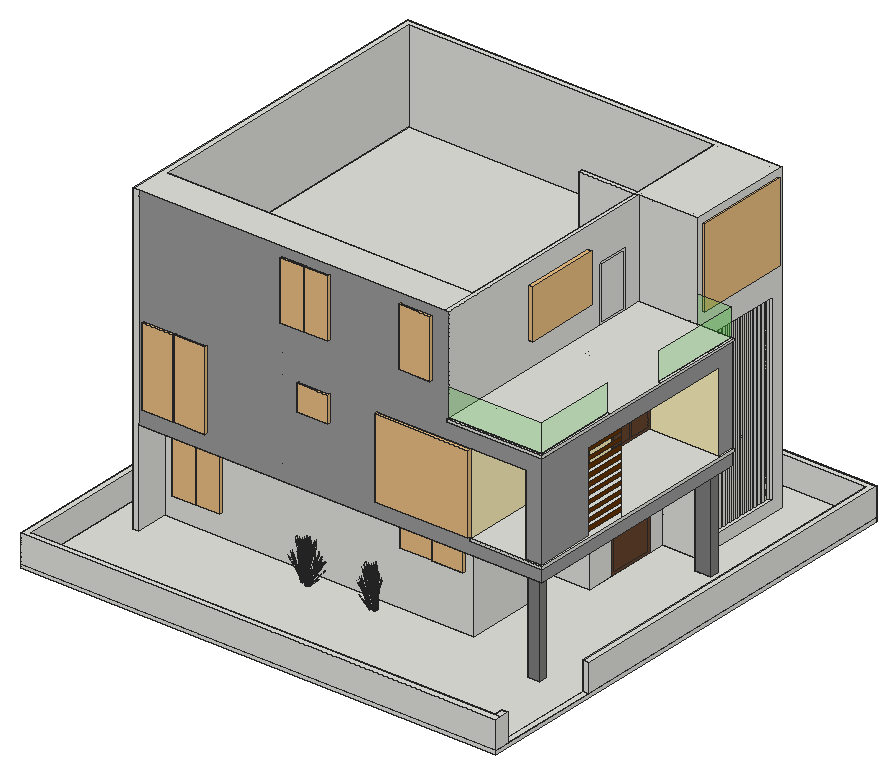
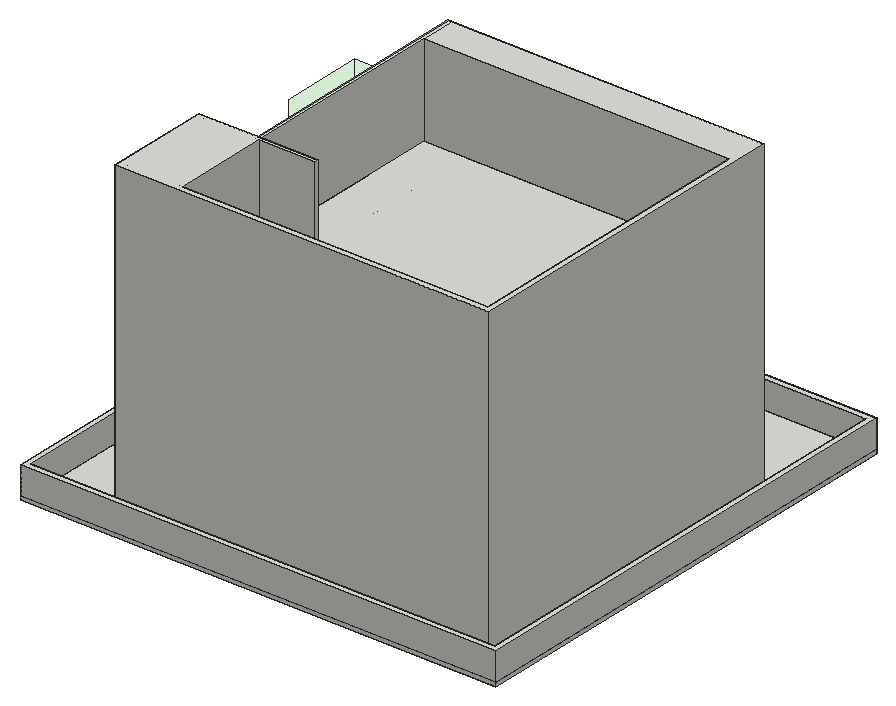
# SketchUp Ruby script. Lengths in millimetres.
U = 1.mm
M = Sketchup.active_model
def pt(a) = Geom::Point3d.new(a.map { |v| v * U })
def face(e, loops, mat)
  f = e.add_face(loops[0].map { |a| pt(a) })
  loops[1..].each { |l| e.add_face(l.map { |a| pt(a) }).erase! }
  f.material = f.back_material = mat if mat
  f
end
# faces: each face lists its corners as indices into pts; further lists are holes
def faces(e, pts, list, mat = nil) = list.each { |f| face(e, (f[0].is_a?(Array) ? f : [f]).map { |l| l.map { |i| pts[i] } }, mat) }
# xy, xz, yz: faces in a plane at the given z, y or x. An outline is a flat list of corners, or four numbers for a rectangle; further outlines are holes
def ring(l) = l.size == 4 ? [[l[0], l[1]], [l[2], l[1]], [l[2], l[3]], [l[0], l[3]]] : l.each_slice(2).to_a
def flat(e, list, mat, &to3) = list.each { |f| face(e, (f[0].is_a?(Array) ? f : [f]).map { |l| ring(l).map { |u, v| to3.(u, v) } }, mat) }
def xy(e, z, list, mat = nil) = flat(e, list, mat) { |x, y| [x, y, z] }
def xz(e, y, list, mat = nil) = flat(e, list, mat) { |x, z| [x, y, z] }
def yz(e, x, list, mat = nil) = flat(e, list, mat) { |y, z| [x, y, z] }
def lines(e, pts, list) = list.each { |a, b| e.add_line(pt(pts[a]), pt(pts[b])) }
# prism: a flat outline (further loops are holes) pulled along v
def prism(e, loops, v, mat = nil)
  f = face(e, loops, mat); d = Geom::Vector3d.new(v.map { |x| x * U })
  f.pushpull(f.normal.samedirection?(d) ? d.length : -d.length)
end
def box(e, o, s, mat = nil) = prism(e, [[o, [o[0] + s[0], o[1], o[2]], [o[0] + s[0], o[1] + s[1], o[2]], [o[0], o[1] + s[1], o[2]]]], [0, 0, s[2]], mat)
def at(x, y, z, deg = 0) = Geom::Transformation.translation(pt([x, y, z])) * Geom::Transformation.rotation(ORIGIN, Z_AXIS, deg.degrees)
def axes(o, x, y, z) = Geom::Transformation.new([*x, 0, *y, 0, *z, 0, *pt(o).to_a, 1])
def part(name) = M.definitions.add(name)
# library, detail: a bought-in or finely detailed component or shape, given as its bounding box
def library(name, o, s) = part(name).tap { |d| box(d.entities, o, s) }
def detail(e, o, s) = box(e.add_group.entities, o, s)
def put(e, d, t, mat = nil) = e.add_instance(d, t).tap { |i| i.material = mat if mat }
def group(e, t, mat = nil) = e.add_group.tap { |g| g.transformation = t; g.material = mat if mat }.entities
root = M.entities
M.materials.add("C08_Toffee_Ember").color = [102, 51, 0]
M.materials.add("D02_Buttercup_Glow").color = [255, 242, 189]
M.materials.add("Glass_Basic_01").color = [75, 255, 58]
M.materials["Glass_Basic_01"].alpha = 0.2
M.materials.add("LightPink_Translucent").color = [144, 107, 117]
M.materials["LightPink_Translucent"].alpha = 0.8
M.materials.add("ThomThom - Waistcoat1").color = [155, 155, 155]
M.materials.add("ThomThom - Waistcoat2").color = [127, 127, 126]
M.materials.add("Wood_Veneer_15_1K").color = [103, 69, 45]
c1 = part("blade")
p = [[54.7,5.3,558.8],[0,4.4,0],[2.3,11.5,0],[55.5,7.8,558.8],[58.2,7.8,558.8],[9.8,11.5,0],
  [62.9,5.7,838.2],[63,6,838.2],[63.4,6,838.2]]
faces(c1.entities,p,[[0,1,2,3],[4,5,2,3],[6,0,3,7],[7,3,4,8]])
c2 = part("seeds")
p = [[7.6,-2.7,35.1],[-0.2,-0.6,40.4],[-0.2,-0.8,0.9],[3.5,-1.8,-1.7],[7.5,-0.8,76.3],[3.7,0.2,78.9]]
faces(c2.entities,p,[[0,1,2,3],[1,0,4,5]],"LightPink_Translucent")
c3 = part("blade with seeds")
put(c3.entities,c1,at(0,0,0))
put(c3.entities,c2,axes([60.9,6.5,787.2],[1.5799,-0.05474,1.17369],[-0.12525,1.92788,0.29478],[-0.07173,-0.02425,1.56792]))
c4 = library("Three-panel window",[0,0,0],[127.5,2149.6,1524])
c5 = library("Group\#4",[0,0,0],[1200.6,88.7,3023])
put(root,c3,axes([7561.3,4255.6,60.5],[-1.54892,-0.2182,0.49198],[0.31522,-1.23236,0.19306],[0.22636,0.119,1.70813]))
put(root,c3,axes([9992.7,4305.7,37.9],[0.03108,0.16322,1.76342],[-0.62654,0.85237,-0.26939],[-0.44504,-0.04296,0.30037]))
put(root,c3,axes([7529.9,4332.9,56],[-0.39985,-0.89288,0],[1.1418,-0.31268,0],[0,0,1.54371]))
put(root,c3,axes([7510.5,4311.4,66.5],[-0.23642,0.92427,0.1448],[-1.15506,-0.16044,-0.41347],[-0.21021,-0.09491,1.26744]))
put(root,c3,axes([10062.4,4383.8,51.5],[-0.28787,-0.90242,-0.30978],[1.14332,-0.25625,0.30978],[-0.23049,-0.10406,1.38974]))
put(root,c3,axes([7567.9,4329.7,55.5],[1.2866,-0.3514,-0.19198],[0.45209,1.01223,0.00008],[0.14202,-0.03884,1.73897]))
put(root,c3,axes([7579.2,4340.5,62.8],[0.35402,-1.02926,0.17642],[1.29548,0.29127,0.35086],[-0.22379,0.00501,1.60407]))
put(root,c3,axes([7571.7,4281.2,56.2],[0.85545,0.66896,0],[-0.85545,0.66896,0],[0,0,1.69266]))
put(root,c3,axes([10099.7,4382.5,62.8],[1.31687,-0.27488,0.17642],[0.32517,1.02297,0.35086],[-0.11745,-0.14905,1.60407]))
put(root,c3,axes([7448.2,4249.3,84.9],[0.34834,-0.14982,1.77064],[0.12012,1.04605,0.13857],[-0.75452,0.1388,0.63284]))
put(root,c3,axes([7630.6,4273.8,62.8],[-0.96285,-0.75439,0.17642],[0.97031,-0.7317,0.35086],[-0.10634,0.15406,1.60407]))
put(root,c3,axes([7585.3,4244.8,52.3],[1.27479,0.1698,-0.62353],[-0.26901,1.04736,-0.16365],[0.38043,0.12691,1.37633]))
put(root,c3,axes([10054.3,4393.7,51.2],[-1.14694,-0.51783,-0.49651],[0.68554,-0.92854,0],[-0.26122,-0.11794,1.57504]))
put(root,c3,axes([7728.4,4291.3,70.2],[-0.75718,0.17097,1.1486],[0.35641,-0.70661,0.84392],[0.40168,0.04835,0.25299]))
put(root,c3,axes([9989.4,4296.3,115],[-1.01846,-0.28891,-0.35414],[0.29705,-0.84289,0.4572],[-0.41005,0.07729,0.87481]))
put(root,c3,axes([7522.7,4343.2,55.8],[-1.23546,-0.46496,0],[0.59459,-0.96613,0],[0,0,1.62707]))
put(root,c3,axes([7548.8,4311.7,62.6],[-1.19666,-0.83357,-0.25192],[1.00694,-0.93603,0.5513],[-0.32224,0.09751,1.68216]))
put(root,c3,axes([7468.8,4352.3,63],[1.14694,0.51783,0.49651],[-0.68554,0.92854,0],[-0.26122,-0.11794,1.57504]))
put(root,c3,axes([10133.5,4347.2,67.7],[-1.23732,0.68758,-0.29095],[-0.8228,-0.97154,-0.50002],[-0.30528,-0.09867,1.59708]))
put(root,c3,axes([7571.5,4261.3,69],[0.59459,-0.93321,0.44739],[1.23546,0.44912,-0.21531],[0,0.21512,1.43643]))
put(root,c3,axes([7565.7,4274.8,58.2],[0,1.19774,-0.05637],[-1.53239,0,0],[0,0.03764,1.79368]))
put(root,c3,axes([7387.2,4263.8,118.9],[-0.332,0.94205,-0.51099],[-1.13828,-0.3229,-0.3958],[-0.45829,0.08638,0.97773]))
put(root,c3,axes([7568.5,4253.3,56.2],[0.73619,0.86927,-0.44739],[-1.11511,0.61213,0.21531],[0.23824,0.10756,1.43643]))
put(root,c3,axes([7695,4346.6,99.8],[-0.23455,-0.87059,-0.03492],[1.10861,-0.20015,-0.15832],[0.23151,0.05519,0.52218]))
put(root,c3,axes([7452,4366.1,60.3],[-0.7662,1.03778,0],[-1.28187,-0.57875,-0.51607],[-0.29196,-0.13181,1.63711]))
put(root,c3,axes([10130.5,4354.9,66.5],[-0.23642,0.92427,0.1448],[-1.15506,-0.16044,-0.41347],[-0.21021,-0.09491,1.26744]))
put(root,c3,axes([7650.7,4274.5,63],[0,-1.03566,0.49651],[1.37109,0,0],[0,0.23588,1.57504]))
put(root,c3,axes([7563.5,4294.2,69],[1.33077,-0.06393,0.44739],[0.12035,1.06125,-0.21531],[-0.23824,0.10756,1.43643]))
put(root,c3,axes([7584.6,4266.7,66.5],[1.1418,-0.30203,0.1448],[0.39985,0.86246,-0.41347],[0,0.18981,1.26744]))
put(root,c3,axes([10199.2,4383.9,62.8],[0.35402,-1.02926,0.17642],[1.29548,0.29127,0.35086],[-0.22379,0.00501,1.60407]))
put(root,c3,axes([7533.4,4307.2,56.2],[-1.33077,0.06393,-0.44739],[-0.12035,-1.06125,0.21531],[-0.23824,0.10756,1.43643]))
put(root,c3,axes([10068.2,4292.7,84.9],[0.34834,-0.14982,1.77064],[0.12012,1.04605,0.13857],[-0.75452,0.1388,0.63284]))
put(root,c3,axes([7692.3,4320.1,65.8],[-0.29514,-0.25472,1.43002],[0.38401,-0.84262,-0.30754],[0.59714,0.11414,0.61141]))
put(root,c3,axes([10142.7,4386.6,55.8],[-1.23546,-0.46496,0],[0.59459,-0.96613,0],[0,0,1.62707]))
put(root,c3,axes([10168.8,4355.2,62.6],[-1.19666,-0.83357,-0.25192],[1.00694,-0.93603,0.5513],[-0.32224,0.09751,1.68216]))
put(root,c3,axes([10088.8,4395.8,63],[1.14694,0.51783,0.49651],[-0.68554,0.92854,0],[-0.26122,-0.11794,1.57504]))
put(root,c3,axes([7558.3,4343.6,56],[1.23546,0.46496,0],[-0.59459,0.96613,0],[0,0,1.74954]))
put(root,c3,axes([7570.9,4369.7,55.7],[-0.75665,-1.04141,-0.05142],[1.28187,-0.57875,0.51607],[-0.31588,0.09915,1.6363]))
put(root,c3,axes([7564,4305.8,66.5],[0.90538,0.62224,0.1448],[-0.75521,0.70202,-0.41347],[-0.21021,0.09491,1.26744]))
put(root,c3,axes([7386.2,4276.1,98.5],[0.42521,-0.21906,1.71376],[0.35798,1.01226,0.13857],[-0.66754,0.22878,0.73262]))
put(root,c3,axes([10007.2,4307.2,118.9],[-0.332,0.94205,-0.51099],[-1.13828,-0.3229,-0.3958],[-0.45829,0.08638,0.97773]))
put(root,c3,axes([10072,4409.5,60.3],[-0.7662,1.03778,0],[-1.28187,-0.57875,-0.51607],[-0.29196,-0.13181,1.63711]))
put(root,c3,axes([10183.5,4337.6,69],[1.33077,-0.06393,0.44739],[0.12035,1.06125,-0.21531],[-0.23824,0.10756,1.43643]))
put(root,c3,axes([7623.5,4333.1,126.5],[1.22504,0.02494,-0.71045],[-0.08228,1.05005,0.08574],[0.51899,0.11081,1.00501]))
put(root,c3,axes([7588.5,4354.5,63],[1.14694,-0.51783,0.49651],[0.68554,0.92854,0],[-0.26122,0.11794,1.57504]))
put(root,c3,axes([10153.4,4350.7,56.2],[-1.33077,0.06393,-0.44739],[-0.12035,-1.06125,0.21531],[-0.23824,0.10756,1.43643]))
put(root,c3,axes([7547.1,4333.7,58.2],[0.53281,1.18979,-0.06012],[-1.52239,0.41691,0],[0.01861,0.04155,1.72173]))
put(root,c3,axes([7562.1,4366.4,51.5],[-1.14332,-0.25625,-0.30978],[0.28787,-0.90242,0.30978],[-0.23049,0.10406,1.38974]))
put(root,c3,axes([7352.5,4319.9,65.8],[0.42589,0.08502,1.43002],[0.2745,0.86839,-0.30754],[-0.57851,0.16255,0.61141]))
put(root,c3,axes([7674.4,4279,60.4],[1.53239,0,0],[0,1.1575,-0.51607],[0,0.26363,1.63711]))
put(root,c3,axes([7658.8,4294.1,55.9],[-1.53164,-0.00828,-0.04976],[0,-1.1575,0.49943],[-0.04813,0.2635,1.58352]))
put(root,c3,axes([7574.6,4268.5,67.7],[1.38012,0.49416,-0.29095],[-0.66454,1.04299,-0.50002],[0.04337,0.25608,1.59708]))
put(root,c3,axes([7330,4366.1,70.2],[0.51072,-0.46938,1.1486],[0.20153,0.74307,0.84392],[-0.36908,0.13305,0.25299]))
put(root,c3,axes([7642.2,4344.1,115],[0.69728,0.64842,-0.35414],[-0.79619,0.61382,0.4572],[0.40453,0.09339,0.87481]))
put(root,c3,axes([7650.7,4298.3,51.5],[-0.85545,0.64616,-0.30978],[-0.85545,-0.64616,0.30978],[0,0.20813,1.38974]))
put(root,c3,axes([7557.1,4299.9,67.7],[0.1428,1.18174,-0.29095],[-1.48733,0.07145,-0.50002],[-0.26191,0.15741,1.59708]))
put(root,c3,axes([10190.8,4413.2,55.7],[-0.75665,-1.04141,-0.05142],[1.28187,-0.57875,0.51607],[-0.31588,0.09915,1.6363]))
put(root,c3,axes([7570.9,4288.2,56.2],[-0.59459,0.93321,-0.44739],[-1.23546,-0.44912,0.21531],[0,0.21512,1.43643]))
put(root,c3,axes([10184,4349.2,66.5],[0.90538,0.62224,0.1448],[-0.75521,0.70202,-0.41347],[-0.21021,0.09491,1.26744]))
put(root,c3,axes([7378.9,4314.6,115],[-1.06674,0.14801,-0.35414],[-0.28168,-0.84611,0.4572],[-0.30569,0.22726,0.87481]))
put(root,c3,axes([10006.2,4319.5,98.5],[0.42521,-0.21906,1.71376],[0.35798,1.01226,0.13857],[-0.66754,0.22878,0.73262]))
put(root,c3,axes([7534.4,4322.9,52.3],[-0.82544,0.77843,-0.62353],[-1.0254,-0.70586,-0.16365],[-0.33076,0.19418,1.37633]))
put(root,c3,axes([10208.5,4397.9,63],[1.14694,-0.51783,0.49651],[0.68554,0.92854,0],[-0.26122,0.11794,1.57504]))
put(root,c3,axes([10182.1,4409.9,51.5],[-1.14332,-0.25625,-0.30978],[0.28787,-0.90242,0.30978],[-0.23049,0.10406,1.38974]))
put(root,c3,axes([7571.7,4356.2,59.2],[1.53422,0.33662,0.30756],[-0.38383,1.20322,-0.36492],[-0.25393,0.15059,1.64885]))
put(root,c3,axes([7568.9,4376.8,51.2],[-1.14694,0.51783,-0.49651],[-0.68554,-0.92854,0],[-0.26122,0.11794,1.57504]))
put(root,c3,axes([7665.7,4298.9,51.2],[0,1.03566,-0.49651],[-1.37109,0,0],[0,0.23588,1.57504]))
put(root,c3,axes([9972.5,4363.4,65.8],[0.42589,0.08502,1.43002],[0.2745,0.86839,-0.30754],[-0.57851,0.16255,0.61141]))
put(root,c3,axes([7578.6,4301.9,98.5],[-0.45521,-0.17844,1.71376],[0.94204,-0.74856,0.13857],[0.58713,0.33769,0.73262]))
put(root,c3,axes([9950,4409.6,70.2],[0.51072,-0.46938,1.1486],[0.20153,0.74307,0.84392],[-0.36908,0.13305,0.25299]))
put(root,c3,axes([7621.4,4353.5,70.2],[-0.69001,-0.29779,1.1486],[0.89096,-0.30257,0.84392],[0.24031,0.2563,0.25299]))
put(root,c3,axes([10177.1,4343.4,67.7],[0.1428,1.18174,-0.29095],[-1.48733,0.07145,-0.50002],[-0.26191,0.15741,1.59708]))
put(root,c3,axes([9998.9,4358,115],[-1.06674,0.14801,-0.35414],[-0.28168,-0.84611,0.4572],[-0.30569,0.22726,0.87481]))
put(root,c3,axes([7425.7,4293.4,98.5],[0.30609,-0.31822,1.71376],[0.77286,0.85893,0.13857],[-0.53009,0.39116,0.73262]))
put(root,c3,axes([7401.3,4317.1,118.9],[0.31482,0.94565,-0.51099],[-1.19224,0.16542,-0.3958],[-0.34166,0.254,0.97773]))
put(root,c3,axes([7595.3,4372.7,60.3],[0.7662,1.03778,0],[-1.28187,0.57875,-0.51607],[-0.29196,0.13181,1.63711]))
put(root,c3,axes([7626.4,4381.6,37.9],[0.08928,-0.14952,1.76342],[1.12407,-0.44035,-0.26939],[0.34078,0.22791,0.30037]))
put(root,c3,axes([7578.8,4268.4,72.2],[-0.03348,-0.97511,1.41272],[1.51511,0.25277,0.59816],[-0.35835,0.53357,1.3335]))
put(root,c3,axes([7588.6,4295.3,53.2],[0.44936,0.94823,-0.69212],[-1.29441,0.3415,-0.18165],[0.04967,0.32109,1.52773]))
put(root,c3,axes([10154.4,4366.3,52.3],[-0.82544,0.77843,-0.62353],[-1.0254,-0.70586,-0.16365],[-0.33076,0.19418,1.37633]))
put(root,c3,axes([7364.1,4378.4,37.9],[0.16438,0.10347,1.76342],[0.27873,0.95868,-0.26939],[-0.36432,0.20444,0.30037]))
put(root,c3,axes([7581.8,4363.9,118.9],[1.20928,-0.24619,-0.51099],[0.21154,0.93233,-0.3958],[0.32481,0.26718,0.97773]))
put(root,c3,axes([10191.7,4399.6,59.2],[1.53422,0.33662,0.30756],[-0.38383,1.20322,-0.36492],[-0.25393,0.15059,1.64885]))
put(root,c3,axes([10188.9,4420.3,51.2],[-1.14694,0.51783,-0.49651],[-0.68554,-0.92854,0],[-0.26122,0.11794,1.57504]))
put(root,c3,axes([7624.2,4387.9,67.7],[-0.78586,-0.03248,1.0506],[0.51898,-0.68985,0.58006],[0.31045,0.24509,0.8241]))
put(root,c3,axes([10045.7,4336.9,98.5],[0.30609,-0.31822,1.71376],[0.77286,0.85893,0.13857],[-0.53009,0.39116,0.73262]))
put(root,c3,axes([10021.3,4360.5,118.9],[0.31482,0.94565,-0.51099],[-1.19224,0.16542,-0.3958],[-0.34166,0.254,0.97773]))
put(root,c3,axes([7419.9,4313.3,98.5],[0.22818,-0.35597,1.71376],[0.95725,0.73667,0.13857],[-0.43183,0.45914,0.73262]))
put(root,c3,axes([10215.3,4416.2,60.3],[0.7662,1.03778,0],[-1.28187,0.57875,-0.51607],[-0.29196,0.13181,1.63711]))
put(root,c3,axes([7559.1,4345.4,65.8],[0.02163,-0.34331,1.43002],[1.03345,-0.38348,-0.30754],[0.31903,0.4109,0.61141]))
put(root,c3,axes([10198.7,4311.8,72.2],[-0.03348,-0.97511,1.41272],[1.51511,0.25277,0.59816],[-0.35835,0.53357,1.3335]))
put(root,c3,axes([9984.1,4421.8,37.9],[0.16438,0.10347,1.76342],[0.27873,0.95868,-0.26939],[-0.36432,0.20444,0.30037]))
put(root,c3,axes([7426.6,4364.3,115],[-0.82919,0.54528,-0.35414],[-0.78493,-0.62262,0.4572],[-0.11943,0.31634,0.87481]))
put(root,c3,axes([7440,4418.1,70.2],[-0.03171,-0.6158,1.1486],[0.7925,0.43922,0.84392],[-0.15586,0.29352,0.25299]))
put(root,c3,axes([7493,4380.8,37.9],[0.19833,-0.05635,1.76342],[1.19302,0.31018,-0.26939],[0.03489,0.3496,0.30037]))
put(root,c3,axes([7447.5,4357.8,127.1],[0.87728,0.69587,-0.5672],[-0.92674,0.60943,-0.43934],[-0.13348,0.35356,1.08528]))
put(root,c3,axes([7423.3,4384.3,71.7],[1.11329,-0.1834,0.06507],[0.25594,0.73887,-0.86304],[-0.07058,0.37403,0.7736]))
put(root,c3,axes([7513.6,4374.9,118.9],[1.20468,0.25962,-0.51099],[-0.41292,0.89013,-0.3958],[0.11046,0.35838,0.97773]))
put(root,c3,axes([7531,4328.2,98.5],[-0.28013,-0.33252,1.71376],[1.29445,-0.27994,0.13857],[0.29256,0.52202,0.73262]))
put(root,c3,axes([10039.9,4356.8,98.5],[0.22818,-0.35597,1.71376],[0.95725,0.73667,0.13857],[-0.43183,0.45914,0.73262]))
put(root,c3,axes([7499.7,4388.8,115],[-0.36946,0.79643,-0.35414],[-1.07787,-0.23229,0.4572],[0.09883,0.32066,0.87481]))
put(root,c3,axes([10046.6,4407.8,115],[-0.82919,0.54528,-0.35414],[-0.78493,-0.62262,0.4572],[-0.11943,0.31634,0.87481]))
put(root,c3,axes([7440.6,4349.7,135.6],[-0.03189,0.95798,-0.7886],[-1.34277,-0.06434,0.09517],[-0.14171,0.40585,1.11556]))
put(root,c3,axes([10060,4461.6,70.2],[-0.03171,-0.6158,1.1486],[0.7925,0.43922,0.84392],[-0.15586,0.29352,0.25299]))
put(root,c3,axes([7472.9,4332.4,98.5],[-0.02999,-0.3975,1.71376],[1.30002,0.26369,0.13857],[-0.08041,0.56647,0.73262]))
put(root,c3,axes([7502.5,4370.6,126.5],[0.5849,0.8421,-0.71045],[-1.20401,0.4693,0.08574],[0.13677,0.40688,1.00501]))
put(root,c3,axes([10067.5,4401.2,127.1],[0.87728,0.69587,-0.5672],[-0.92674,0.60943,-0.43934],[-0.13348,0.35356,1.08528]))
put(root,c3,axes([7416.5,4404.3,65.8],[0.38672,-0.16338,1.43002],[0.95481,0.49262,-0.30754],[-0.28419,0.42626,0.61141]))
put(root,c3,axes([10043.3,4427.8,71.7],[1.11329,-0.1834,0.06507],[0.25594,0.73887,-0.86304],[-0.07058,0.37403,0.7736]))
put(root,c3,axes([10060.6,4393.1,135.6],[-0.03189,0.95798,-0.7886],[-1.34277,-0.06434,0.09517],[-0.14171,0.40585,1.11556]))
put(root,c3,axes([10092.9,4375.9,98.5],[-0.02999,-0.3975,1.71376],[1.30002,0.26369,0.13857],[-0.08041,0.56647,0.73262]))
put(root,c3,axes([7429.2,4384,85.4],[0.02693,-0.53464,1.54345],[1.21102,0.2824,0.21329],[-0.10493,0.5698,0.72882]))
put(root,c3,axes([10036.5,4447.7,65.8],[0.38672,-0.16338,1.43002],[0.95481,0.49262,-0.30754],[-0.28419,0.42626,0.61141]))
put(root,c3,axes([10049.2,4427.4,85.4],[0.02693,-0.53464,1.54345],[1.21102,0.2824,0.21329],[-0.10493,0.5698,0.72882]))
g1 = group(root,at(0,0,-152.4))
xy(g1,0,[[0,0,18288,18288]])
xy(g1,152.4,[[228.6,228.6,18059.4,18059.4],[18059.4,562.7,18288,4460.6]])
xy(g1,1219.2,[[0,0,18288,0,18288,228.6,228.6,228.6,228.6,18059.4,18059.4,18059.4,18059.4,4460.6,18288,4460.6,18288,18288,0,18288],[18059.4,228.6,18288,562.7]])
xz(g1,0,[[0,0,18288,1219.2]])
xz(g1,228.6,[[228.6,152.4,18059.4,1219.2]])
xz(g1,562.7,[[18059.4,152.4,18288,1219.2]])
xz(g1,4460.6,[[18059.4,152.4,18288,1219.2]])
xz(g1,18059.4,[[228.6,152.4,18059.4,1219.2]])
xz(g1,18288,[[0,0,18288,1219.2]])
yz(g1,0,[[0,0,18288,1219.2]])
yz(g1,228.6,[[228.6,152.4,18059.4,1219.2]])
yz(g1,18059.4,[[228.6,152.4,562.7,1219.2],[4460.6,152.4,11604.7,1219.2],[11604.7,152.4,18059.4,1219.2]])
yz(g1,18288,[[0,0,18288,0,18288,1219.2,4460.6,1219.2,4460.6,152.4,562.7,152.4,562.7,1219.2,0,1219.2]])
g2 = group(root,at(0,0,0))
xy(g2,0,[[1295.4,3810,1524,3810,1524,5029.2,13411.2,5029.2,13411.2,5181.6,1524,5181.6,1524,16764,14173.2,16764,14173.2,9448.8,14325.6,9448.8,14325.6,16764,15392.4,16764,15392.4,12954,15544.8,12954,15544.8,16992.6,1295.4,16992.6],[16230.6,4114.8,16687.8,4419.6],[11646.4,5181.6,13411.2,7620],[11646.4,7620,13411.2,7772.4],[12528.8,7772.4,12681.2,9448.8],
  [11646.4,9448.8,14173.2,9601.2],[16078.2,12344.4,16687.8,12649.2],[14325.6,12954,15392.4,16764],[15544.8,12954,15697.2,16992.6]])
xy(g2,76.2,[[9744.7,10591.8,14325.6,12268.2]])
xy(g2,457.2,[[15544.8,13411.2,15697.2,16535.4]])
xy(g2,2971.8,[[9744.7,10591.8,14325.6,12268.2]])
xy(g2,3657.6,[[[1524,3810,1524,5029.2,13411.2,5029.2,13411.2,7772.4,12681.2,7772.4,12681.2,9448.8,14325.6,9448.8,14325.6,12954,16992.6,12954,16992.6,3810],[16078.2,12344.4,16687.8,12649.2],[16230.6,4114.8,16687.8,4419.6]],[11646.4,5029.2,13411.2,7620],[11646.4,7620,13411.2,7772.4],[11646.4,7772.4,12528.8,9448.8]])
xy(g2,4165.6,[[14306.8,3733.8,16992.6,3810],[16992.6,3733.8,17068.8,12954]])
xy(g2,4267.2,[[14306.8,3733.8,14325.6,3810],[[14325.6,3733.8,17068.8,12344.4],[16383,3810,16992.6,6056.6]],[16383,3810,16992.6,6056.6],[16992.6,12344.4,17068.8,12954]])
xy(g2,7315.2,[[14325.6,3810,14325.6,12344.4,16992.6,12344.4,16992.6,6056.6,16383,6056.6,16383,3810]])
xy(g2,7467.6,[[15544.8,13411.2,15697.2,16535.4]])
xy(g2,7924.8,[[14325.6,12954,15392.4,16764]])
xy(g2,7975.6,[[13411.2,3733.8,17068.8,3810],[16992.6,3810,17068.8,7010.7],[16992.6,7010.7,17068.8,12954]])
xy(g2,8077.2,[[13411.2,3733.8,17068.8,3810],[13411.2,3810,16992.6,3810,16992.6,7010.7,17068.8,7010.7,17068.8,9449.1,16992.6,9449.1,16992.6,12954,13411.2,12954],[16992.6,3810,17068.8,7010.7],[13258.8,7772.4,13411.2,9448.8],[11646.4,9448.8,13258.8,9601.2],
  [13258.8,9448.8,13411.2,9601.2],[16992.6,9449.1,17068.8,12954],[13258.8,9601.2,13411.2,12801.6],[13258.8,12801.6,13411.2,12801.6,13411.2,12954,15392.4,12954,15392.4,13106.4,13411.2,13106.4,13411.2,16764,13258.8,16764,13258.8,13106.4,11125.2,13106.4,11125.2,12954,13258.8,12954],[13411.2,13106.4,15392.4,16764]])
xy(g2,8229.6,[[1524,5181.6,13258.8,5181.6,13258.8,12954,11125.2,12954,11125.2,13106.4,12882.9,13106.4,13258.8,14172,13258.8,16764,1524,16764]])
xy(g2,11734.8,[[1295.4,3810,13258.8,3810,13258.8,5181.6,1524,5181.6,1524,16764,13258.8,16764,13258.8,12954,15697.2,12954,15697.2,16992.6,1295.4,16992.6],[13258.8,3810,13411.2,3810,13411.2,12954,13258.8,12954,13258.8,13106.4,11125.2,13106.4,11125.2,12954,13258.8,12954]])
xz(g2,3733.8,[[14306.8,4165.6,17068.8,4267.2],[13411.2,7975.6,17068.8,8077.2]])
xz(g2,3810,[[1295.4,0,1524,11734.8]])
xz(g2,3810,[[13411.2,8077.2,16992.6,9144]],"Glass_Basic_01")
xz(g2,3810,[[1524,3657.6,16992.6,3657.6,16992.6,4165.6,14306.8,4165.6,14306.8,4267.2,10668,4267.2,10668,7315.2,16383,7315.2,16383,4267.2,16992.6,4267.2,16992.6,7975.6,13411.2,7975.6,13411.2,11734.8,1524,11734.8]],"ThomThom - Waistcoat1")
xz(g2,3810,[[10668,4267.2,14325.6,7315.2]],"ThomThom - Waistcoat2")
xz(g2,4114.8,[[16230.6,0,16687.8,3657.6]],"ThomThom - Waistcoat2")
xz(g2,4419.6,[[16230.6,0,16687.8,3657.6]])
xz(g2,5029.2,[[1524,0,13411.2,3657.6],[7010.4,3657.6,13411.2,8077.2]])
xz(g2,5181.6,[[1524,0,11646.4,3657.6],[1524,3657.6,11646.4,8229.6],[1524,8229.6,13258.8,11734.8]])
xz(g2,6056.6,[[16383,4267.2,16992.6,7315.2]])
xz(g2,7772.4,[[11646.4,0,12528.8,3657.6],[12528.8,0,12681.2,3657.6],[12681.2,0,13411.2,3657.6]])
xz(g2,9448.8,[[11646.4,0,12528.8,3657.6],[12528.8,0,12681.2,0,12681.2,3657.6,14173.2,3657.6,14173.2,4871.6,11646.4,4871.6,11646.4,3657.6,12528.8,3657.6],[12681.2,0,14325.6,3657.6],[14173.2,3657.6,14325.6,4871.6]])
xz(g2,10591.8,[[9744.7,76.2,14325.6,2971.8]])
xz(g2,12268.2,[[9744.7,76.2,14325.6,2971.8]])
xz(g2,12344.4,[[14325.6,4267.2,16992.6,7315.2]],"D02_Buttercup_Glow")
xz(g2,12344.4,[[16078.2,0,16687.8,3657.6]],"ThomThom - Waistcoat2")
xz(g2,12649.2,[[16078.2,0,16687.8,3657.6]],"ThomThom - Waistcoat2")
xz(g2,12954,[[14325.6,0,15697.2,3657.6],[14325.6,3657.6,15392.4,7924.8],[15392.4,3657.6,15697.2,8077.2],[15697.2,3657.6,15697.2,8077.2,17068.8,8077.2,17068.8,7975.6,16992.6,7975.6,16992.6,4267.2,17068.8,4267.2,17068.8,4165.6,16992.6,4165.6,16992.6,3657.6],[11125.2,8077.2,12829.1,8229.6],
  [12829.1,8077.2,13258.8,8229.6],[13411.2,8077.2,15697.2,11734.8],[11125.2,8229.6,13258.8,11734.8]])
xz(g2,12954,[[15697.2,8077.2,16992.6,9144]],"Glass_Basic_01")
xz(g2,13106.4,[[11125.2,8077.2,12882.9,8229.6],[12882.9,8077.2,12882.9,8229.6,11125.2,8229.6,11125.2,11734.8,13258.8,11734.8,13258.8,8077.2]])
xz(g2,13411.2,[[15544.8,457.2,15697.2,7467.6]])
xz(g2,16535.4,[[15544.8,457.2,15697.2,7467.6]])
xz(g2,16764,[[14325.6,0,15392.4,7924.8],[1524,8229.6,13258.8,11734.8]])
xz(g2,16992.6,[[1295.4,0,15697.2,11734.8]])
yz(g2,1295.4,[[3810,0,16992.6,11734.8]])
yz(g2,1524,[[3810,0,5029.2,3657.6],[5181.6,0,16764,8229.6],[5181.6,8229.6,16764,11734.8]])
yz(g2,11125.2,[[12954,8077.2,13106.4,8229.6],[12954,8229.6,13106.4,11734.8]])
yz(g2,11646.4,[[5181.6,0,7620,3657.6],[7620,0,7772.4,3657.6]])
yz(g2,12528.8,[[7772.4,0,9448.8,3657.6]])
yz(g2,12681.2,[[7772.4,0,9448.8,3657.6]])
yz(g2,13258.8,[[7772.4,8077.2,9448.8,8229.6],[9448.8,8077.2,9601.2,8229.6],[9601.2,8077.2,12801.6,8229.6],[12801.6,8077.2,12954,8229.6],[13106.4,8077.2,13106.4,11734.8,16764,11734.8,16764,8229.6,14172,8229.6,14172,8077.2],
  [14172,8077.2,16764,8229.6],[5181.6,8229.6,12954,11734.8]])
yz(g2,13411.2,[[5029.2,0,7772.4,3657.6],[3733.8,7975.6,3810,8077.2],[3810,8077.2,11082.7,8077.2,11082.7,10210.8,12301.9,10210.8,12301.9,8077.2,12954,8077.2,12954,11734.8,3810,11734.8],[[11082.7,8077.2,12301.9,10210.8],[11133.5,8128,12251.1,10160]],[11133.5,8128,12251.1,10160]])
yz(g2,14306.8,[[3733.8,4165.6,3810,4267.2]])
yz(g2,14325.6,[[9448.8,0,10515.6,0,10515.6,3048,12344.4,3048,12344.4,0,12954,0,12954,3657.6,9448.8,3657.6],[12954,0,16764,7924.8],[7645.4,4292.6,9423.4,4546.6],[7645.4,4597.4,9423.4,4851.4],[7645.4,4902.2,9423.4,5156.2],
  [7645.4,5207,9423.4,5461],[7645.4,5511.8,9423.4,5765.8],[7645.4,5816.6,9423.4,6070.6],[7645.4,6121.4,9423.4,6375.4],[7645.4,6426.2,9423.4,6680.2],
  [7645.4,6731,9423.4,6985]])
yz(g2,14325.6,[[3810,4267.2,7620,4267.2,7620,7010.4,9448.8,7010.4,9448.8,4267.2,10515.6,4267.2,10515.6,7315.2,3810,7315.2]],"D02_Buttercup_Glow")
yz(g2,14325.6,[[[10515.6,0,12344.4,3048],[10591.8,76.2,12268.2,2971.8]],[10591.8,76.2,12268.2,2971.8],[[7620,4267.2,9448.8,4572],[7645.4,4292.6,9423.4,4546.6]],[[10515.6,4267.2,12344.4,7315.2],[11455.4,4343.4,12268.2,7239],[10591.8,4343.4,11404.6,7239]],[10591.8,4343.4,11404.6,7239],
  [11455.4,4343.4,12268.2,7239],[[7620,4572,9448.8,4876.8],[7645.4,4597.4,9423.4,4851.4]],[[7620,4876.8,9448.8,5181.6],[7645.4,4902.2,9423.4,5156.2]],[[7620,5181.6,9448.8,5486.4],[7645.4,5207,9423.4,5461]],[[7620,5486.4,9448.8,5791.2],[7645.4,5511.8,9423.4,5765.8]],
  [[7620,5791.2,9448.8,6096],[7645.4,5816.6,9423.4,6070.6]],[[7620,6096,9448.8,6400.8],[7645.4,6121.4,9423.4,6375.4]],[[7620,6400.8,9448.8,6705.6],[7645.4,6426.2,9423.4,6680.2]],[[7620,6705.6,9448.8,7010.4],[7645.4,6731,9423.4,6985]]],"Wood_Veneer_15_1K")
yz(g2,15392.4,[[12954,7315.2,13106.4,7924.8],[12954,7924.8,13106.4,8077.2],[13106.4,7924.8,16764,8077.2]])
yz(g2,15544.8,[[13411.2,457.2,13473.7,7467.6],[13473.7,457.2,13536.2,7467.6],[13536.2,457.2,13598.7,7467.6],[13598.7,457.2,13661.1,7467.6],[13661.1,457.2,13723.6,7467.6],
  [13723.6,457.2,13786.1,7467.6],[13786.1,457.2,13848.6,7467.6],[13848.6,457.2,13911.1,7467.6],[13911.1,457.2,13973.6,7467.6],[13973.6,457.2,14036,7467.6],
  [14036,457.2,14098.5,7467.6],[14098.5,457.2,14161,7467.6],[14161,457.2,14223.5,7467.6],[14223.5,457.2,14286,7467.6],[14286,457.2,14348.5,7467.6],
  [14348.5,457.2,14410.9,7467.6],[14410.9,457.2,14473.4,7467.6],[14473.4,457.2,14535.9,7467.6],[14535.9,457.2,14598.4,7467.6],[14598.4,457.2,14660.9,7467.6],
  [14660.9,457.2,14723.4,7467.6],[14723.4,457.2,14785.8,7467.6],[14785.8,457.2,14848.3,7467.6],[14848.3,457.2,14910.8,7467.6],[14910.8,457.2,14973.3,7467.6],
  [14973.3,457.2,15035.8,7467.6],[15035.8,457.2,15098.3,7467.6],[15098.3,457.2,15160.8,7467.6],[15160.8,457.2,15223.2,7467.6],[15223.2,457.2,15285.7,7467.6],
  [15285.7,457.2,15348.2,7467.6],[15348.2,457.2,15410.7,7467.6],[15410.7,457.2,15473.2,7467.6],[15473.2,457.2,15535.7,7467.6],[15535.7,457.2,15598.1,7467.6],
  [15598.1,457.2,15660.6,7467.6],[15660.6,457.2,15723.1,7467.6],[15723.1,457.2,15785.6,7467.6],[15785.6,457.2,15848.1,7467.6],[15848.1,457.2,15910.6,7467.6],
  [15910.6,457.2,15973,7467.6],[15973,457.2,16035.5,7467.6],[16035.5,457.2,16098,7467.6],[16098,457.2,16160.5,7467.6],[16160.5,457.2,16223,7467.6],
  [16223,457.2,16285.5,7467.6],[16285.5,457.2,16347.9,7467.6],[16347.9,457.2,16410.4,7467.6],[16410.4,457.2,16472.9,7467.6],[16472.9,457.2,16535.4,7467.6]])
yz(g2,15697.2,[[[12954,0,16992.6,11734.8],[13411.2,457.2,16535.4,7467.6]]])
yz(g2,16078.2,[[12344.4,0,12649.2,3657.6]],"ThomThom - Waistcoat2")
yz(g2,16230.6,[[4114.8,0,4419.6,3657.6]],"ThomThom - Waistcoat2")
yz(g2,16383,[[3810,4267.2,6056.6,7315.2]])
yz(g2,16687.8,[[4114.8,0,4419.6,3657.6],[12344.4,0,12649.2,3657.6]],"ThomThom - Waistcoat2")
yz(g2,16992.6,[[6056.6,4419.6,7630.6,4572],[6056.6,4724.4,7630.6,4876.8],[6056.6,5029.2,7630.6,5181.6],[6056.6,5334,7630.6,5486.4],[6056.6,5638.8,7630.6,5791.2],
  [6056.6,5943.6,7630.6,6096],[6056.6,6248.4,7630.6,6400.8],[6056.6,6553.2,7630.6,6705.6],[6056.6,6858,7630.6,7010.4],[6056.6,7162.8,7630.6,7315.2]],"C08_Toffee_Ember")
yz(g2,16992.6,[[3810,8077.2,7010.7,9144],[9449.1,8077.2,12954,9144]],"Glass_Basic_01")
yz(g2,16992.6,[[3810,3657.6,12954,4165.6],[3810,4267.2,6056.6,4267.2,6056.6,7315.2,12344.4,7315.2,12344.4,4267.2,12954,4267.2,12954,7975.6,3810,7975.6]],"ThomThom - Waistcoat1")
yz(g2,17068.8,[[3733.8,4165.6,12954,4267.2],[3733.8,7975.6,12954,8077.2]])
p = [[18059.4,228.6,0],[18059.4,18059.4,0],[228.6,18059.4,0],[228.6,228.6,0],[18288,0,0],[18288,18288,0],
  [0,18288,0],[0,0,0],[15392.4,13106.4,3657.6],[15544.8,13106.4,3657.6],[15392.4,13106.4,7315.2],[15544.8,13106.4,7924.8],
  [7010.4,5029.2,7315.2],[7010.4,5181.6,7924.8],[14173.2,9601.2,7769.6],[14173.2,9448.8,7769.6],[14173.2,9601.2,0],[14173.2,9448.8,8077.2],
  [14173.2,5181.6,3657.6],[14173.2,5181.6,8077.2],[13411.2,16764,11734.8],[13411.2,16764,8077.2],[15392.4,16764,8077.2],[15392.4,16764,11734.8],
  [13411.2,13106.4,11734.8],[13411.2,13106.4,8077.2],[15392.4,13106.4,11734.8],[15392.4,13106.4,8077.2],[14173.2,7772.4,7769.6],[14173.2,9448.8,4871.6],
  [14173.2,9601.2,8077.2],[11646.4,9601.2,8077.2],[11646.4,9601.2,8229.6],[11646.4,9448.8,8077.2],[11646.4,9448.8,8229.6],[14325.6,9448.8,8077.2],
  [14325.6,9448.8,7315.2],[11646.4,9448.8,7924.8],[11646.4,9448.8,7769.6],[11646.4,7772.4,3657.6],[11646.4,7772.4,8229.6],[11646.4,9448.8,4871.6],
  [7010.4,3810,7315.2],[7010.4,5029.2,8077.2],[7010.4,3810,8077.2],[7010.4,5029.2,4267.2],[7010.4,3810,4267.2],[12801.6,3810,10363.2],
  [12801.6,3810,9144],[16992.6,7630.6,7162.8],[16992.6,7630.6,7010.4],[16992.6,7630.6,6858],[16992.6,7630.6,6705.6],[16992.6,7630.6,6553.2],
  [16992.6,7630.6,6400.8],[16992.6,7630.6,6248.4],[16992.6,7630.6,6096],[16992.6,7630.6,5943.6],[16992.6,7630.6,5791.2],[16992.6,7630.6,5638.8],
  [16992.6,7630.6,5486.4],[16992.6,7630.6,5334],[16992.6,7630.6,5181.6],[16992.6,7630.6,5029.2],[16992.6,7630.6,4876.8],[16992.6,7630.6,4724.4],
  [16992.6,7630.6,4572],[16992.6,7630.6,4419.6],[16992.6,7630.6,4267.2]]
lines(g2,p,[[0,1],[1,2],[2,3],[3,0],[4,5],[5,6],[6,7],[7,4],[8,9],[10,11],[12,13],[14,15],
  [14,16],[15,17],[18,19],[20,21],[22,23],[24,25],[26,27],[28,15],[15,29],[14,30],[31,32],[33,34],
  [35,36],[37,33],[38,37],[39,40],[41,38],[12,42],[43,44],[45,46],[47,48],[49,50],[51,52],[53,54],
  [55,56],[57,58],[59,60],[61,62],[63,64],[65,66],[67,68]])
put(g2,c4,axes([14269.9,3682.5,4277.3],[0,1,0],[-1.6756,0,0],[0,0,1.9836]))
put(g2,c4,axes([15793.7,16751.6,8467.1],[-1,0,0],[0,-1.6756,0],[0,0,1.9836]))
put(g2,c4,axes([13602.3,10472.1,9087.6],[-2.34429,0,0],[0,-1.32372,0],[0,0,1.23217]))
put(g2,c5,axes([11588.6,3721.3,9144],[1,0,0],[0,1,0],[0,0,0.74]))
put(g2,c5,axes([7654,3721.3,6303.9],[1,0,0],[0,1,0],[0,0,0.32271]))
put(g2,c5,axes([1705.9,3721.3,4277.3],[1,0,0],[0,1,0],[0,0,0.99312]))
put(g2,c5,axes([2925.1,3721.3,4277.3],[1,0,0],[0,1,0],[0,0,0.99312]))
put(g2,c5,axes([7928.5,3721.3,9144],[0.76,0,0],[0,1,0],[0,0,0.74]))
put(g2,c5,axes([7016,3716.3,9144],[0.76,0,0],[0,1,0],[0,0,0.74]))
put(g2,c5,axes([11873.8,4945.5,2120.7],[1,0,0],[0,1,0],[0,0,0.32271]))
put(g2,c5,axes([10654.5,4945.5,2120.7],[1,0,0],[0,1,0],[0,0,0.32271]))
put(g2,c5,axes([1882.9,4940.5,842.7],[0.76,0,0],[0,1,0],[0,0,0.74]))
put(g2,c5,axes([2795.3,4945.5,842.7],[0.76,0,0],[0,1,0],[0,0,0.74]))
put(g2,c5,axes([12917.3,9360.1,1285.3],[1,0,0],[0,1,0],[0,0,0.49276]))
